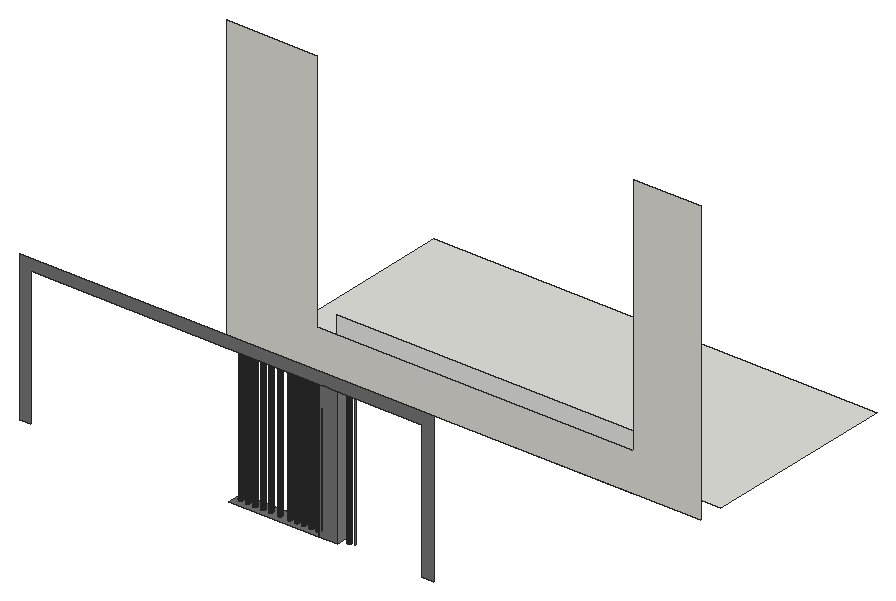
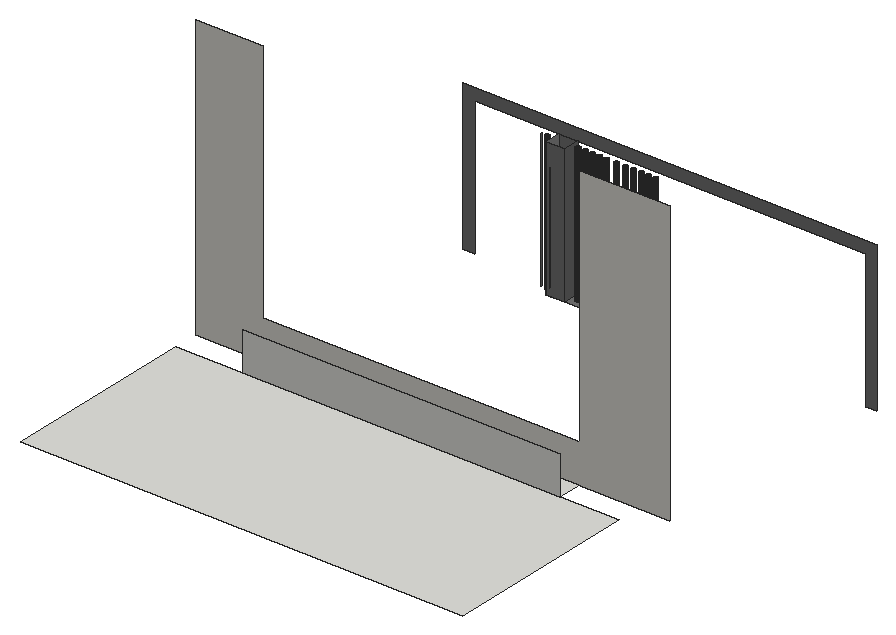
# SketchUp Ruby script. Lengths in inches.
U = 1.inch
M = Sketchup.active_model
def pt(a) = Geom::Point3d.new(a.map { |v| v * U })
def face(e, loops, mat)
  f = e.add_face(loops[0].map { |a| pt(a) })
  loops[1..].each { |l| e.add_face(l.map { |a| pt(a) }).erase! }
  f.material = f.back_material = mat if mat
  f
end
# faces: each face lists its corners as indices into pts; further lists are holes
def faces(e, pts, list, mat = nil) = list.each { |f| face(e, (f[0].is_a?(Array) ? f : [f]).map { |l| l.map { |i| pts[i] } }, mat) }
# xy, xz, yz: faces in a plane at the given z, y or x. An outline is a flat list of corners, or four numbers for a rectangle; further outlines are holes
def ring(l) = l.size == 4 ? [[l[0], l[1]], [l[2], l[1]], [l[2], l[3]], [l[0], l[3]]] : l.each_slice(2).to_a
def flat(e, list, mat, &to3) = list.each { |f| face(e, (f[0].is_a?(Array) ? f : [f]).map { |l| ring(l).map { |u, v| to3.(u, v) } }, mat) }
def xy(e, z, list, mat = nil) = flat(e, list, mat) { |x, y| [x, y, z] }
def xz(e, y, list, mat = nil) = flat(e, list, mat) { |x, z| [x, y, z] }
def yz(e, x, list, mat = nil) = flat(e, list, mat) { |y, z| [x, y, z] }
def lines(e, pts, list) = list.each { |a, b| e.add_line(pt(pts[a]), pt(pts[b])) }
# prism: a flat outline (further loops are holes) pulled along v
def prism(e, loops, v, mat = nil)
  f = face(e, loops, mat); d = Geom::Vector3d.new(v.map { |x| x * U })
  f.pushpull(f.normal.samedirection?(d) ? d.length : -d.length)
end
def box(e, o, s, mat = nil) = prism(e, [[o, [o[0] + s[0], o[1], o[2]], [o[0] + s[0], o[1] + s[1], o[2]], [o[0], o[1] + s[1], o[2]]]], [0, 0, s[2]], mat)
def at(x, y, z, deg = 0) = Geom::Transformation.translation(pt([x, y, z])) * Geom::Transformation.rotation(ORIGIN, Z_AXIS, deg.degrees)
def axes(o, x, y, z) = Geom::Transformation.new([*x, 0, *y, 0, *z, 0, *pt(o).to_a, 1])
def part(name) = M.definitions.add(name)
# library, detail: a bought-in or finely detailed component or shape, given as its bounding box
def library(name, o, s) = part(name).tap { |d| box(d.entities, o, s) }
def detail(e, o, s) = box(e.add_group.entities, o, s)
def put(e, d, t, mat = nil) = e.add_instance(d, t).tap { |i| i.material = mat if mat }
def group(e, t, mat = nil) = e.add_group.tap { |g| g.transformation = t; g.material = mat if mat }.entities
root = M.entities
M.materials.add("[Color M04]").color = [142, 142, 142]
M.materials.add("[Color M05]").color = [114, 114, 114]
M.materials.add("[Terrazzo Tile Light]").color = [219, 217, 210]
xy(root,9,[[151.04,291.34,388.47,309.84],[107.23,309.84,438.59,455.8]])
xy(root,17.125,[[285.42,125.1875,299.8,137.375],[222.24,129.51,221.84,129.56,221.46,129.72,221.13,129.97,220.89,130.29,220.73,130.67,220.68,131.07,220.73,131.48,220.89,131.86,221.13,132.18,221.46,132.43,221.84,132.58,222.24,132.64,222.64,132.58,223.02,132.43,223.34,132.18,223.59,131.86,223.75,131.48,223.8,131.07,223.75,130.67,223.59,130.29,223.34,129.97,223.02,129.72,222.64,129.56],[227.8,129.51,227.4,129.56,227.02,129.72,226.7,129.97,226.45,130.29,226.29,130.67,226.24,131.07,226.29,131.48,226.45,131.86,226.7,132.18,227.02,132.43,227.4,132.58,227.8,132.64,228.21,132.58,228.58,132.43,228.91,132.18,229.16,131.86,229.3125,131.48,229.36,131.07,229.3125,130.67,229.16,130.29,228.91,129.97,228.58,129.72,228.21,129.56],[233.24,129.51,232.84,129.56,232.46,129.72,232.13,129.97,231.89,130.29,231.73,130.67,231.68,131.07,231.73,131.48,231.89,131.86,232.13,132.18,232.46,132.43,232.84,132.58,233.24,132.64,233.64,132.58,234.02,132.43,234.34,132.18,234.59,131.86,234.75,131.48,234.8,131.07,234.75,130.67,234.59,130.29,234.34,129.97,234.02,129.72,233.64,129.56],[239.24,129.51,238.84,129.56,238.46,129.72,238.13,129.97,237.89,130.29,237.73,130.67,237.68,131.07,237.73,131.48,237.89,131.86,238.13,132.18,238.46,132.43,238.84,132.58,239.24,132.64,239.64,132.58,240.02,132.43,240.34,132.18,240.59,131.86,240.75,131.48,240.8,131.07,240.75,130.67,240.59,130.29,240.34,129.97,240.02,129.72,239.64,129.56],
  [244.99,129.51,244.59,129.56,244.21,129.72,243.88,129.97,243.64,130.29,243.48,130.67,243.43,131.07,243.48,131.48,243.64,131.86,243.88,132.18,244.21,132.43,244.59,132.58,244.99,132.64,245.39,132.58,245.77,132.43,246.09,132.18,246.34,131.86,246.5,131.48,246.55,131.07,246.5,130.67,246.34,130.29,246.09,129.97,245.77,129.72,245.39,129.56],[251.86,129.51,251.46,129.56,251.08,129.72,250.76,129.97,250.51,130.29,250.36,130.67,250.3,131.07,250.36,131.48,250.51,131.86,250.76,132.18,251.08,132.43,251.46,132.58,251.86,132.64,252.27,132.58,252.65,132.43,252.97,132.18,253.22,131.86,253.375,131.48,253.43,131.07,253.375,130.67,253.22,130.29,252.97,129.97,252.65,129.72,252.27,129.56],[259.18,129.51,258.77,129.56,258.4,129.72,258.07,129.97,257.82,130.29,257.67,130.67,257.61,131.07,257.67,131.48,257.82,131.86,258.07,132.18,258.4,132.43,258.77,132.58,259.18,132.64,259.58,132.58,259.96,132.43,260.28,132.18,260.53,131.86,260.6875,131.48,260.74,131.07,260.6875,130.67,260.53,130.29,260.28,129.97,259.96,129.72,259.58,129.56],[264.74,129.51,264.34,129.56,263.96,129.72,263.63,129.97,263.39,130.29,263.23,130.67,263.18,131.07,263.23,131.48,263.39,131.86,263.63,132.18,263.96,132.43,264.34,132.58,264.74,132.64,265.14,132.58,265.52,132.43,265.84,132.18,266.09,131.86,266.25,131.48,266.3,131.07,266.25,130.67,266.09,130.29,265.84,129.97,265.52,129.72,265.14,129.56],[269.74,129.51,269.34,129.56,268.96,129.72,268.63,129.97,268.39,130.29,268.23,130.67,268.18,131.07,268.23,131.48,268.39,131.86,268.63,132.18,268.96,132.43,269.34,132.58,269.74,132.64,270.14,132.58,270.52,132.43,270.84,132.18,271.09,131.86,271.25,131.48,271.3,131.07,271.25,130.67,271.09,130.29,270.84,129.97,270.52,129.72,270.14,129.56],
  [275.43,129.51,275.02,129.56,274.65,129.72,274.32,129.97,274.07,130.29,273.92,130.67,273.86,131.07,273.92,131.48,274.07,131.86,274.32,132.18,274.65,132.43,275.02,132.58,275.43,132.64,275.83,132.58,276.21,132.43,276.53,132.18,276.78,131.86,276.9375,131.48,276.99,131.07,276.9375,130.67,276.78,130.29,276.53,129.97,276.21,129.72,275.83,129.56],[280.86,129.51,280.46,129.56,280.08,129.72,279.76,129.97,279.51,130.29,279.36,130.67,279.3,131.07,279.36,131.48,279.51,131.86,279.76,132.18,280.08,132.43,280.46,132.58,280.86,132.64,281.27,132.58,281.65,132.43,281.97,132.18,282.22,131.86,282.375,131.48,282.43,131.07,282.375,130.67,282.22,130.29,281.97,129.97,281.65,129.72,281.27,129.56],[303.86,129.51,303.46,129.56,303.08,129.72,302.76,129.97,302.51,130.29,302.36,130.67,302.3,131.07,302.36,131.48,302.51,131.86,302.76,132.18,303.08,132.43,303.46,132.58,303.86,132.64,304.27,132.58,304.65,132.43,304.97,132.18,305.22,131.86,305.375,131.48,305.43,131.07,305.375,130.67,305.22,130.29,304.97,129.97,304.65,129.72,304.27,129.56]])
xy(root,17.125,[[[217.93,125.1875,285.42,137.375],[222.24,129.51,221.84,129.56,221.46,129.72,221.13,129.97,220.89,130.29,220.73,130.67,220.68,131.07,220.73,131.48,220.89,131.86,221.13,132.18,221.46,132.43,221.84,132.58,222.24,132.64,222.64,132.58,223.02,132.43,223.34,132.18,223.59,131.86,223.75,131.48,223.8,131.07,223.75,130.67,223.59,130.29,223.34,129.97,223.02,129.72,222.64,129.56],[280.86,129.51,280.46,129.56,280.08,129.72,279.76,129.97,279.51,130.29,279.36,130.67,279.3,131.07,279.36,131.48,279.51,131.86,279.76,132.18,280.08,132.43,280.46,132.58,280.86,132.64,281.27,132.58,281.65,132.43,281.97,132.18,282.22,131.86,282.375,131.48,282.43,131.07,282.375,130.67,282.22,130.29,281.97,129.97,281.65,129.72,281.27,129.56],[227.8,129.51,227.4,129.56,227.02,129.72,226.7,129.97,226.45,130.29,226.29,130.67,226.24,131.07,226.29,131.48,226.45,131.86,226.7,132.18,227.02,132.43,227.4,132.58,227.8,132.64,228.21,132.58,228.58,132.43,228.91,132.18,229.16,131.86,229.3125,131.48,229.36,131.07,229.3125,130.67,229.16,130.29,228.91,129.97,228.58,129.72,228.21,129.56],[275.43,129.51,275.02,129.56,274.65,129.72,274.32,129.97,274.07,130.29,273.92,130.67,273.86,131.07,273.92,131.48,274.07,131.86,274.32,132.18,274.65,132.43,275.02,132.58,275.43,132.64,275.83,132.58,276.21,132.43,276.53,132.18,276.78,131.86,276.9375,131.48,276.99,131.07,276.9375,130.67,276.78,130.29,276.53,129.97,276.21,129.72,275.83,129.56],[233.24,129.51,232.84,129.56,232.46,129.72,232.13,129.97,231.89,130.29,231.73,130.67,231.68,131.07,231.73,131.48,231.89,131.86,232.13,132.18,232.46,132.43,232.84,132.58,233.24,132.64,233.64,132.58,234.02,132.43,234.34,132.18,234.59,131.86,234.75,131.48,234.8,131.07,234.75,130.67,234.59,130.29,234.34,129.97,234.02,129.72,233.64,129.56],[269.74,129.51,269.34,129.56,268.96,129.72,268.63,129.97,268.39,130.29,268.23,130.67,268.18,131.07,268.23,131.48,268.39,131.86,268.63,132.18,268.96,132.43,269.34,132.58,269.74,132.64,270.14,132.58,270.52,132.43,270.84,132.18,271.09,131.86,271.25,131.48,271.3,131.07,271.25,130.67,271.09,130.29,270.84,129.97,270.52,129.72,270.14,129.56],[239.24,129.51,238.84,129.56,238.46,129.72,238.13,129.97,237.89,130.29,237.73,130.67,237.68,131.07,237.73,131.48,237.89,131.86,238.13,132.18,238.46,132.43,238.84,132.58,239.24,132.64,239.64,132.58,240.02,132.43,240.34,132.18,240.59,131.86,240.75,131.48,240.8,131.07,240.75,130.67,240.59,130.29,240.34,129.97,240.02,129.72,239.64,129.56],[264.74,129.51,264.34,129.56,263.96,129.72,263.63,129.97,263.39,130.29,263.23,130.67,263.18,131.07,263.23,131.48,263.39,131.86,263.63,132.18,263.96,132.43,264.34,132.58,264.74,132.64,265.14,132.58,265.52,132.43,265.84,132.18,266.09,131.86,266.25,131.48,266.3,131.07,266.25,130.67,266.09,130.29,265.84,129.97,265.52,129.72,265.14,129.56],[244.99,129.51,244.59,129.56,244.21,129.72,243.88,129.97,243.64,130.29,243.48,130.67,243.43,131.07,243.48,131.48,243.64,131.86,243.88,132.18,244.21,132.43,244.59,132.58,244.99,132.64,245.39,132.58,245.77,132.43,246.09,132.18,246.34,131.86,246.5,131.48,246.55,131.07,246.5,130.67,246.34,130.29,246.09,129.97,245.77,129.72,245.39,129.56],[259.18,129.51,258.77,129.56,258.4,129.72,258.07,129.97,257.82,130.29,257.67,130.67,257.61,131.07,257.67,131.48,257.82,131.86,258.07,132.18,258.4,132.43,258.77,132.58,259.18,132.64,259.58,132.58,259.96,132.43,260.28,132.18,260.53,131.86,260.6875,131.48,260.74,131.07,260.6875,130.67,260.53,130.29,260.28,129.97,259.96,129.72,259.58,129.56],[251.86,129.51,251.46,129.56,251.08,129.72,250.76,129.97,250.51,130.29,250.36,130.67,250.3,131.07,250.36,131.48,250.51,131.86,250.76,132.18,251.08,132.43,251.46,132.58,251.86,132.64,252.27,132.58,252.65,132.43,252.97,132.18,253.22,131.86,253.375,131.48,253.43,131.07,253.375,130.67,253.22,130.29,252.97,129.97,252.65,129.72,252.27,129.56]]],"[Color M05]")
xz(root,125.1875,[[61.88,17.125,69.95,17.125,69.95,119.59,362.74,119.59,362.74,17.125,371.37,17.125,371.37,128.625,61.88,128.625],[285.42,17.125,299.8,119.59]],"[Color M05]")
xz(root,137.375,[[285.42,17.125,299.8,119.59]],"[Color M05]")
xz(root,291.34,[[83.3125,9,438.59,9,438.59,220,388.47,220,388.47,38.0625,151.04,38.0625,151.04,220,83.3125,220]],"[Terrazzo Tile Light]")
xz(root,309.84,[[151.04,9,388.47,38.0625]])
yz(root,285.42,[[125.1875,17.125,137.375,119.59]],"[Color M05]")
yz(root,299.8,[[125.1875,17.125,137.375,119.59]],"[Color M04]")
p = [[222.24,129.51,17.125],[222.64,129.56,17.125],[222.64,129.56,119.59],[222.24,129.51,119.59],[227.4,129.56,17.125],[227.8,129.51,17.125],
  [227.8,129.51,119.59],[227.4,129.56,119.59],[228.21,129.56,17.125],[228.21,129.56,119.59],[232.84,129.56,17.125],[233.24,129.51,17.125],
  [233.24,129.51,119.59],[232.84,129.56,119.59],[233.64,129.56,17.125],[233.64,129.56,119.59],[238.84,129.56,17.125],[239.24,129.51,17.125],
  [239.24,129.51,119.59],[238.84,129.56,119.59],[239.64,129.56,17.125],[239.64,129.56,119.59],[244.59,129.56,17.125],[244.99,129.51,17.125],
  [244.99,129.51,119.59],[244.59,129.56,119.59],[245.39,129.56,17.125],[245.39,129.56,119.59],[251.46,129.56,17.125],[251.86,129.51,17.125],
  [251.86,129.51,119.59],[251.46,129.56,119.59],[252.27,129.56,17.125],[252.27,129.56,119.59],[258.77,129.56,17.125],[259.18,129.51,17.125],
  [259.18,129.51,119.59],[258.77,129.56,119.59],[259.58,129.56,17.125],[259.58,129.56,119.59],[264.34,129.56,17.125],[264.74,129.51,17.125],
  [264.74,129.51,119.59],[264.34,129.56,119.59],[265.14,129.56,17.125],[265.14,129.56,119.59],[269.34,129.56,17.125],[269.74,129.51,17.125],
  [269.74,129.51,119.59],[269.34,129.56,119.59],[270.14,129.56,17.125],[270.14,129.56,119.59],[275.02,129.56,17.125],[275.43,129.51,17.125],
  [275.43,129.51,119.59],[275.02,129.56,119.59],[275.83,129.56,17.125],[275.83,129.56,119.59],[280.46,129.56,17.125],[280.86,129.51,17.125],
  [280.86,129.51,119.59],[280.46,129.56,119.59],[281.27,129.56,17.125],[281.27,129.56,119.59],[303.46,129.56,17.125],[303.86,129.51,17.125],
  [303.86,129.51,119.59],[303.46,129.56,119.59],[304.27,129.56,17.125],[304.27,129.56,119.59],[223.02,129.72,17.125],[223.02,129.72,119.59],
  [227.02,129.72,17.125],[227.02,129.72,119.59],[228.58,129.72,17.125],[228.58,129.72,119.59],[232.46,129.72,17.125],[232.46,129.72,119.59],
  [234.02,129.72,17.125],[234.02,129.72,119.59],[238.46,129.72,17.125],[238.46,129.72,119.59],[240.02,129.72,17.125],[240.02,129.72,119.59],
  [244.21,129.72,17.125],[244.21,129.72,119.59],[245.77,129.72,17.125],[245.77,129.72,119.59],[251.08,129.72,17.125],[251.08,129.72,119.59],
  [252.65,129.72,17.125],[252.65,129.72,119.59],[258.4,129.72,17.125],[258.4,129.72,119.59],[259.96,129.72,17.125],[259.96,129.72,119.59],
  [263.96,129.72,17.125],[263.96,129.72,119.59],[265.52,129.72,17.125],[265.52,129.72,119.59],[268.96,129.72,17.125],[268.96,129.72,119.59],
  [270.52,129.72,17.125],[270.52,129.72,119.59],[274.65,129.72,17.125],[274.65,129.72,119.59],[276.21,129.72,17.125],[276.21,129.72,119.59],
  [280.08,129.72,17.125],[280.08,129.72,119.59],[281.65,129.72,17.125],[281.65,129.72,119.59],[303.08,129.72,17.125],[303.08,129.72,119.59],
  [304.65,129.72,17.125],[304.65,129.72,119.59],[223.34,129.97,17.125],[223.34,129.97,119.59],[226.7,129.97,17.125],[226.7,129.97,119.59],
  [228.91,129.97,17.125],[228.91,129.97,119.59],[232.13,129.97,17.125],[232.13,129.97,119.59],[234.34,129.97,17.125],[234.34,129.97,119.59],
  [238.13,129.97,17.125],[238.13,129.97,119.59],[240.34,129.97,17.125],[240.34,129.97,119.59],[243.88,129.97,17.125],[243.88,129.97,119.59],
  [246.09,129.97,17.125],[246.09,129.97,119.59],[250.76,129.97,17.125],[250.76,129.97,119.59],[252.97,129.97,17.125],[252.97,129.97,119.59],
  [258.07,129.97,17.125],[258.07,129.97,119.59],[260.28,129.97,17.125],[260.28,129.97,119.59],[263.63,129.97,17.125],[263.63,129.97,119.59],
  [265.84,129.97,17.125],[265.84,129.97,119.59],[268.63,129.97,17.125],[268.63,129.97,119.59],[270.84,129.97,17.125],[270.84,129.97,119.59],
  [274.32,129.97,17.125],[274.32,129.97,119.59],[276.53,129.97,17.125],[276.53,129.97,119.59],[279.76,129.97,17.125],[279.76,129.97,119.59],
  [281.97,129.97,17.125],[281.97,129.97,119.59],[302.76,129.97,17.125],[302.76,129.97,119.59],[304.97,129.97,17.125],[304.97,129.97,119.59],
  [223.59,130.29,17.125],[223.59,130.29,119.59],[226.45,130.29,17.125],[226.45,130.29,119.59],[229.16,130.29,17.125],[229.16,130.29,119.59],
  [231.89,130.29,17.125],[231.89,130.29,119.59],[234.59,130.29,17.125],[234.59,130.29,119.59],[237.89,130.29,17.125],[237.89,130.29,119.59],
  [240.59,130.29,17.125],[240.59,130.29,119.59],[243.64,130.29,17.125],[243.64,130.29,119.59],[246.34,130.29,17.125],[246.34,130.29,119.59],
  [250.51,130.29,17.125],[250.51,130.29,119.59],[253.22,130.29,17.125],[253.22,130.29,119.59],[257.82,130.29,17.125],[257.82,130.29,119.59],
  [260.53,130.29,17.125],[260.53,130.29,119.59],[263.39,130.29,17.125],[263.39,130.29,119.59],[266.09,130.29,17.125],[266.09,130.29,119.59],
  [268.39,130.29,17.125],[268.39,130.29,119.59],[271.09,130.29,17.125],[271.09,130.29,119.59],[274.07,130.29,17.125],[274.07,130.29,119.59],
  [276.78,130.29,17.125],[276.78,130.29,119.59],[279.51,130.29,17.125],[279.51,130.29,119.59],[282.22,130.29,17.125],[282.22,130.29,119.59],
  [302.51,130.29,17.125],[302.51,130.29,119.59],[305.22,130.29,17.125],[305.22,130.29,119.59],[223.75,130.67,17.125],[223.75,130.67,119.59],
  [226.29,130.67,17.125],[226.29,130.67,119.59],[229.3125,130.67,17.125],[229.3125,130.67,119.59],[231.73,130.67,17.125],[231.73,130.67,119.59],
  [234.75,130.67,17.125],[234.75,130.67,119.59],[237.73,130.67,17.125],[237.73,130.67,119.59],[240.75,130.67,17.125],[240.75,130.67,119.59],
  [243.48,130.67,17.125],[243.48,130.67,119.59],[246.5,130.67,17.125],[246.5,130.67,119.59],[250.36,130.67,17.125],[250.36,130.67,119.59],
  [253.375,130.67,17.125],[253.375,130.67,119.59],[257.67,130.67,17.125],[257.67,130.67,119.59],[260.6875,130.67,17.125],[260.6875,130.67,119.59],
  [263.23,130.67,17.125],[263.23,130.67,119.59],[266.25,130.67,17.125],[266.25,130.67,119.59],[268.23,130.67,17.125],[268.23,130.67,119.59],
  [271.25,130.67,17.125],[271.25,130.67,119.59],[273.92,130.67,17.125],[273.92,130.67,119.59],[276.9375,130.67,17.125],[276.9375,130.67,119.59],
  [279.36,130.67,17.125],[279.36,130.67,119.59],[282.375,130.67,17.125],[282.375,130.67,119.59],[302.36,130.67,17.125],[302.36,130.67,119.59],
  [305.375,130.67,17.125],[305.375,130.67,119.59],[223.8,131.07,17.125],[223.8,131.07,119.59],[226.24,131.07,17.125],[226.24,131.07,119.59],
  [229.36,131.07,17.125],[229.36,131.07,119.59],[231.68,131.07,17.125],[231.68,131.07,119.59],[234.8,131.07,17.125],[234.8,131.07,119.59],
  [237.68,131.07,17.125],[237.68,131.07,119.59],[240.8,131.07,17.125],[240.8,131.07,119.59],[243.43,131.07,17.125],[243.43,131.07,119.59],
  [246.55,131.07,17.125],[246.55,131.07,119.59],[250.3,131.07,17.125],[250.3,131.07,119.59],[253.43,131.07,17.125],[253.43,131.07,119.59],
  [257.61,131.07,17.125],[257.61,131.07,119.59],[260.74,131.07,17.125],[260.74,131.07,119.59],[263.18,131.07,17.125],[263.18,131.07,119.59],
  [266.3,131.07,17.125],[266.3,131.07,119.59],[268.18,131.07,17.125],[268.18,131.07,119.59],[271.3,131.07,17.125],[271.3,131.07,119.59],
  [273.86,131.07,17.125],[273.86,131.07,119.59],[276.99,131.07,17.125],[276.99,131.07,119.59],[279.3,131.07,17.125],[279.3,131.07,119.59],
  [282.43,131.07,17.125],[282.43,131.07,119.59],[302.3,131.07,17.125],[302.3,131.07,119.59],[305.43,131.07,17.125],[305.43,131.07,119.59],
  [223.75,131.48,17.125],[223.75,131.48,119.59],[226.29,131.48,17.125],[226.29,131.48,119.59],[229.3125,131.48,17.125],[229.3125,131.48,119.59],
  [231.73,131.48,17.125],[231.73,131.48,119.59],[234.75,131.48,17.125],[234.75,131.48,119.59],[237.73,131.48,17.125],[237.73,131.48,119.59],
  [240.75,131.48,17.125],[240.75,131.48,119.59],[243.48,131.48,17.125],[243.48,131.48,119.59],[246.5,131.48,17.125],[246.5,131.48,119.59],
  [250.36,131.48,17.125],[250.36,131.48,119.59],[253.375,131.48,17.125],[253.375,131.48,119.59],[257.67,131.48,17.125],[257.67,131.48,119.59],
  [260.6875,131.48,17.125],[260.6875,131.48,119.59],[263.23,131.48,17.125],[263.23,131.48,119.59],[266.25,131.48,17.125],[266.25,131.48,119.59],
  [268.23,131.48,17.125],[268.23,131.48,119.59],[271.25,131.48,17.125],[271.25,131.48,119.59],[273.92,131.48,17.125],[273.92,131.48,119.59],
  [276.9375,131.48,17.125],[276.9375,131.48,119.59],[279.36,131.48,17.125],[279.36,131.48,119.59],[282.375,131.48,17.125],[282.375,131.48,119.59],
  [302.36,131.48,17.125],[302.36,131.48,119.59],[305.375,131.48,17.125],[305.375,131.48,119.59],[308.17,131.48,17.125],[308.11,131.07,17.125],
  [308.11,131.07,119.59],[308.17,131.48,119.59],[223.59,131.86,17.125],[223.59,131.86,119.59],[226.45,131.86,17.125],[226.45,131.86,119.59],
  [229.16,131.86,17.125],[229.16,131.86,119.59],[231.89,131.86,17.125],[231.89,131.86,119.59],[234.59,131.86,17.125],[234.59,131.86,119.59],
  [237.89,131.86,17.125],[237.89,131.86,119.59],[240.59,131.86,17.125],[240.59,131.86,119.59],[243.64,131.86,17.125],[243.64,131.86,119.59],
  [246.34,131.86,17.125],[246.34,131.86,119.59],[250.51,131.86,17.125],[250.51,131.86,119.59],[253.22,131.86,17.125],[253.22,131.86,119.59],
  [257.82,131.86,17.125],[257.82,131.86,119.59],[260.53,131.86,17.125],[260.53,131.86,119.59],[263.39,131.86,17.125],[263.39,131.86,119.59],
  [266.09,131.86,17.125],[266.09,131.86,119.59],[268.39,131.86,17.125],[268.39,131.86,119.59],[271.09,131.86,17.125],[271.09,131.86,119.59],
  [274.07,131.86,17.125],[274.07,131.86,119.59],[276.78,131.86,17.125],[276.78,131.86,119.59],[279.51,131.86,17.125],[279.51,131.86,119.59],
  [282.22,131.86,17.125],[282.22,131.86,119.59],[302.51,131.86,17.125],[302.51,131.86,119.59],[305.22,131.86,17.125],[305.22,131.86,119.59],
  [223.34,132.18,17.125],[223.34,132.18,119.59],[226.7,132.18,17.125],[226.7,132.18,119.59],[228.91,132.18,17.125],[228.91,132.18,119.59],
  [232.13,132.18,17.125],[232.13,132.18,119.59],[234.34,132.18,17.125],[234.34,132.18,119.59],[238.13,132.18,17.125],[238.13,132.18,119.59],
  [240.34,132.18,17.125],[240.34,132.18,119.59],[243.88,132.18,17.125],[243.88,132.18,119.59],[246.09,132.18,17.125],[246.09,132.18,119.59],
  [250.76,132.18,17.125],[250.76,132.18,119.59],[252.97,132.18,17.125],[252.97,132.18,119.59],[258.07,132.18,17.125],[258.07,132.18,119.59],
  [260.28,132.18,17.125],[260.28,132.18,119.59],[263.63,132.18,17.125],[263.63,132.18,119.59],[265.84,132.18,17.125],[265.84,132.18,119.59],
  [268.63,132.18,17.125],[268.63,132.18,119.59],[270.84,132.18,17.125],[270.84,132.18,119.59],[274.32,132.18,17.125],[274.32,132.18,119.59],
  [276.53,132.18,17.125],[276.53,132.18,119.59],[279.76,132.18,17.125],[279.76,132.18,119.59],[281.97,132.18,17.125],[281.97,132.18,119.59],
  [302.76,132.18,17.125],[302.76,132.18,119.59],[304.97,132.18,17.125],[304.97,132.18,119.59],[223.02,132.43,17.125],[223.02,132.43,119.59],
  [227.02,132.43,17.125],[227.02,132.43,119.59],[228.58,132.43,17.125],[228.58,132.43,119.59],[232.46,132.43,17.125],[232.46,132.43,119.59],
  [234.02,132.43,17.125],[234.02,132.43,119.59],[238.46,132.43,17.125],[238.46,132.43,119.59],[240.02,132.43,17.125],[240.02,132.43,119.59],
  [244.21,132.43,17.125],[244.21,132.43,119.59],[245.77,132.43,17.125],[245.77,132.43,119.59],[251.08,132.43,17.125],[251.08,132.43,119.59],
  [252.65,132.43,17.125],[252.65,132.43,119.59],[258.4,132.43,17.125],[258.4,132.43,119.59],[259.96,132.43,17.125],[259.96,132.43,119.59],
  [263.96,132.43,17.125],[263.96,132.43,119.59],[265.52,132.43,17.125],[265.52,132.43,119.59],[268.96,132.43,17.125],[268.96,132.43,119.59],
  [270.52,132.43,17.125],[270.52,132.43,119.59],[274.65,132.43,17.125],[274.65,132.43,119.59],[276.21,132.43,17.125],[276.21,132.43,119.59],
  [280.08,132.43,17.125],[280.08,132.43,119.59],[281.65,132.43,17.125],[281.65,132.43,119.59],[303.08,132.43,17.125],[303.08,132.43,119.59],
  [304.65,132.43,17.125],[304.65,132.43,119.59],[222.64,132.58,17.125],[222.64,132.58,119.59],[227.4,132.58,17.125],[227.4,132.58,119.59],
  [228.21,132.58,17.125],[228.21,132.58,119.59],[232.84,132.58,17.125],[232.84,132.58,119.59],[233.64,132.58,17.125],[233.64,132.58,119.59],
  [238.84,132.58,17.125],[238.84,132.58,119.59],[239.64,132.58,17.125],[239.64,132.58,119.59],[244.59,132.58,17.125],[244.59,132.58,119.59],
  [245.39,132.58,17.125],[245.39,132.58,119.59],[251.46,132.58,17.125],[251.46,132.58,119.59],[252.27,132.58,17.125],[252.27,132.58,119.59],
  [258.77,132.58,17.125],[258.77,132.58,119.59],[259.58,132.58,17.125],[259.58,132.58,119.59],[264.34,132.58,17.125],[264.34,132.58,119.59],
  [265.14,132.58,17.125],[265.14,132.58,119.59],[269.34,132.58,17.125],[269.34,132.58,119.59],[270.14,132.58,17.125],[270.14,132.58,119.59],
  [275.02,132.58,17.125],[275.02,132.58,119.59],[275.83,132.58,17.125],[275.83,132.58,119.59],[280.46,132.58,17.125],[280.46,132.58,119.59],
  [281.27,132.58,17.125],[281.27,132.58,119.59],[303.46,132.58,17.125],[303.46,132.58,119.59],[304.27,132.58,17.125],[304.27,132.58,119.59],
  [222.24,132.64,17.125],[222.24,132.64,119.59],[227.8,132.64,17.125],[227.8,132.64,119.59],[233.24,132.64,17.125],[233.24,132.64,119.59],
  [239.24,132.64,17.125],[239.24,132.64,119.59],[244.99,132.64,17.125],[244.99,132.64,119.59],[251.86,132.64,17.125],[251.86,132.64,119.59],
  [259.18,132.64,17.125],[259.18,132.64,119.59],[264.74,132.64,17.125],[264.74,132.64,119.59],[269.74,132.64,17.125],[269.74,132.64,119.59],
  [275.43,132.64,17.125],[275.43,132.64,119.59],[280.86,132.64,17.125],[280.86,132.64,119.59],[303.86,132.64,17.125],[303.86,132.64,119.59]]
faces(root,p,[[0,1,2,3],[4,5,6,7],[5,8,9,6],[10,11,12,13],[11,14,15,12],[16,17,18,19],[17,20,21,18],[22,23,24,25],
  [23,26,27,24],[28,29,30,31],[29,32,33,30],[34,35,36,37],[35,38,39,36],[40,41,42,43],[41,44,45,42],[46,47,48,49],
  [47,50,51,48],[52,53,54,55],[53,56,57,54],[58,59,60,61],[59,62,63,60],[64,65,66,67],[65,68,69,66],[1,70,71,2],
  [72,4,7,73],[8,74,75,9],[76,10,13,77],[14,78,79,15],[80,16,19,81],[20,82,83,21],[84,22,25,85],[26,86,87,27],
  [88,28,31,89],[32,90,91,33],[92,34,37,93],[38,94,95,39],[96,40,43,97],[44,98,99,45],[100,46,49,101],[50,102,103,51],
  [104,52,55,105],[56,106,107,57],[108,58,61,109],[62,110,111,63],[112,64,67,113],[68,114,115,69],[70,116,117,71],[118,72,73,119],
  [74,120,121,75],[122,76,77,123],[78,124,125,79],[126,80,81,127],[82,128,129,83],[130,84,85,131],[86,132,133,87],[134,88,89,135],
  [90,136,137,91],[138,92,93,139],[94,140,141,95],[142,96,97,143],[98,144,145,99],[146,100,101,147],[102,148,149,103],[150,104,105,151],
  [106,152,153,107],[154,108,109,155],[110,156,157,111],[158,112,113,159],[114,160,161,115],[116,162,163,117],[164,118,119,165],[120,166,167,121],
  [168,122,123,169],[124,170,171,125],[172,126,127,173],[128,174,175,129],[176,130,131,177],[132,178,179,133],[180,134,135,181],[136,182,183,137],
  [184,138,139,185],[140,186,187,141],[188,142,143,189],[144,190,191,145],[192,146,147,193],[148,194,195,149],[196,150,151,197],[152,198,199,153],
  [200,154,155,201],[156,202,203,157],[204,158,159,205],[160,206,207,161],[162,208,209,163],[210,164,165,211],[166,212,213,167],[214,168,169,215],
  [170,216,217,171],[218,172,173,219],[174,220,221,175],[222,176,177,223],[178,224,225,179],[226,180,181,227],[182,228,229,183],[230,184,185,231],
  [186,232,233,187],[234,188,189,235],[190,236,237,191],[238,192,193,239],[194,240,241,195],[242,196,197,243],[198,244,245,199],[246,200,201,247],
  [202,248,249,203],[250,204,205,251],[206,252,253,207],[208,254,255,209],[256,210,211,257],[212,258,259,213],[260,214,215,261],[216,262,263,217],
  [264,218,219,265],[220,266,267,221],[268,222,223,269],[224,270,271,225],[272,226,227,273],[228,274,275,229],[276,230,231,277],[232,278,279,233],
  [280,234,235,281],[236,282,283,237],[284,238,239,285],[240,286,287,241],[288,242,243,289],[244,290,291,245],[292,246,247,293],[248,294,295,249],
  [296,250,251,297],[252,298,299,253],[254,300,301,255],[302,256,257,303],[258,304,305,259],[306,260,261,307],[262,308,309,263],[310,264,265,311],
  [266,312,313,267],[314,268,269,315],[270,316,317,271],[318,272,273,319],[274,320,321,275],[322,276,277,323],[278,324,325,279],[326,280,281,327],
  [282,328,329,283],[330,284,285,331],[286,332,333,287],[334,288,289,335],[290,336,337,291],[338,292,293,339],[294,340,341,295],[342,296,297,343],
  [298,344,345,299],[346,347,348,349],[300,350,351,301],[352,302,303,353],[304,354,355,305],[356,306,307,357],[308,358,359,309],[360,310,311,361],
  [312,362,363,313],[364,314,315,365],[316,366,367,317],[368,318,319,369],[320,370,371,321],[372,322,323,373],[324,374,375,325],[376,326,327,377],
  [328,378,379,329],[380,330,331,381],[332,382,383,333],[384,334,335,385],[336,386,387,337],[388,338,339,389],[340,390,391,341],[392,342,343,393],
  [344,394,395,345],[350,396,397,351],[398,352,353,399],[354,400,401,355],[402,356,357,403],[358,404,405,359],[406,360,361,407],[362,408,409,363],
  [410,364,365,411],[366,412,413,367],[414,368,369,415],[370,416,417,371],[418,372,373,419],[374,420,421,375],[422,376,377,423],[378,424,425,379],
  [426,380,381,427],[382,428,429,383],[430,384,385,431],[386,432,433,387],[434,388,389,435],[390,436,437,391],[438,392,393,439],[394,440,441,395],
  [396,442,443,397],[444,398,399,445],[400,446,447,401],[448,402,403,449],[404,450,451,405],[452,406,407,453],[408,454,455,409],[456,410,411,457],
  [412,458,459,413],[460,414,415,461],[416,462,463,417],[464,418,419,465],[420,466,467,421],[468,422,423,469],[424,470,471,425],[472,426,427,473],
  [428,474,475,429],[476,430,431,477],[432,478,479,433],[480,434,435,481],[436,482,483,437],[484,438,439,485],[440,486,487,441],[442,488,489,443],
  [490,444,445,491],[446,492,493,447],[494,448,449,495],[450,496,497,451],[498,452,453,499],[454,500,501,455],[502,456,457,503],[458,504,505,459],
  [506,460,461,507],[462,508,509,463],[510,464,465,511],[466,512,513,467],[514,468,469,515],[470,516,517,471],[518,472,473,519],[474,520,521,475],
  [522,476,477,523],[478,524,525,479],[526,480,481,527],[482,528,529,483],[530,484,485,531],[486,532,533,487],[488,534,535,489],[536,490,491,537],
  [492,536,537,493],[538,494,495,539],[496,538,539,497],[540,498,499,541],[500,540,541,501],[542,502,503,543],[504,542,543,505],[544,506,507,545],
  [508,544,545,509],[546,510,511,547],[512,546,547,513],[548,514,515,549],[516,548,549,517],[550,518,519,551],[520,550,551,521],[552,522,523,553],
  [524,552,553,525],[554,526,527,555],[528,554,555,529],[556,530,531,557],[532,556,557,533]],"[Color M05]")
